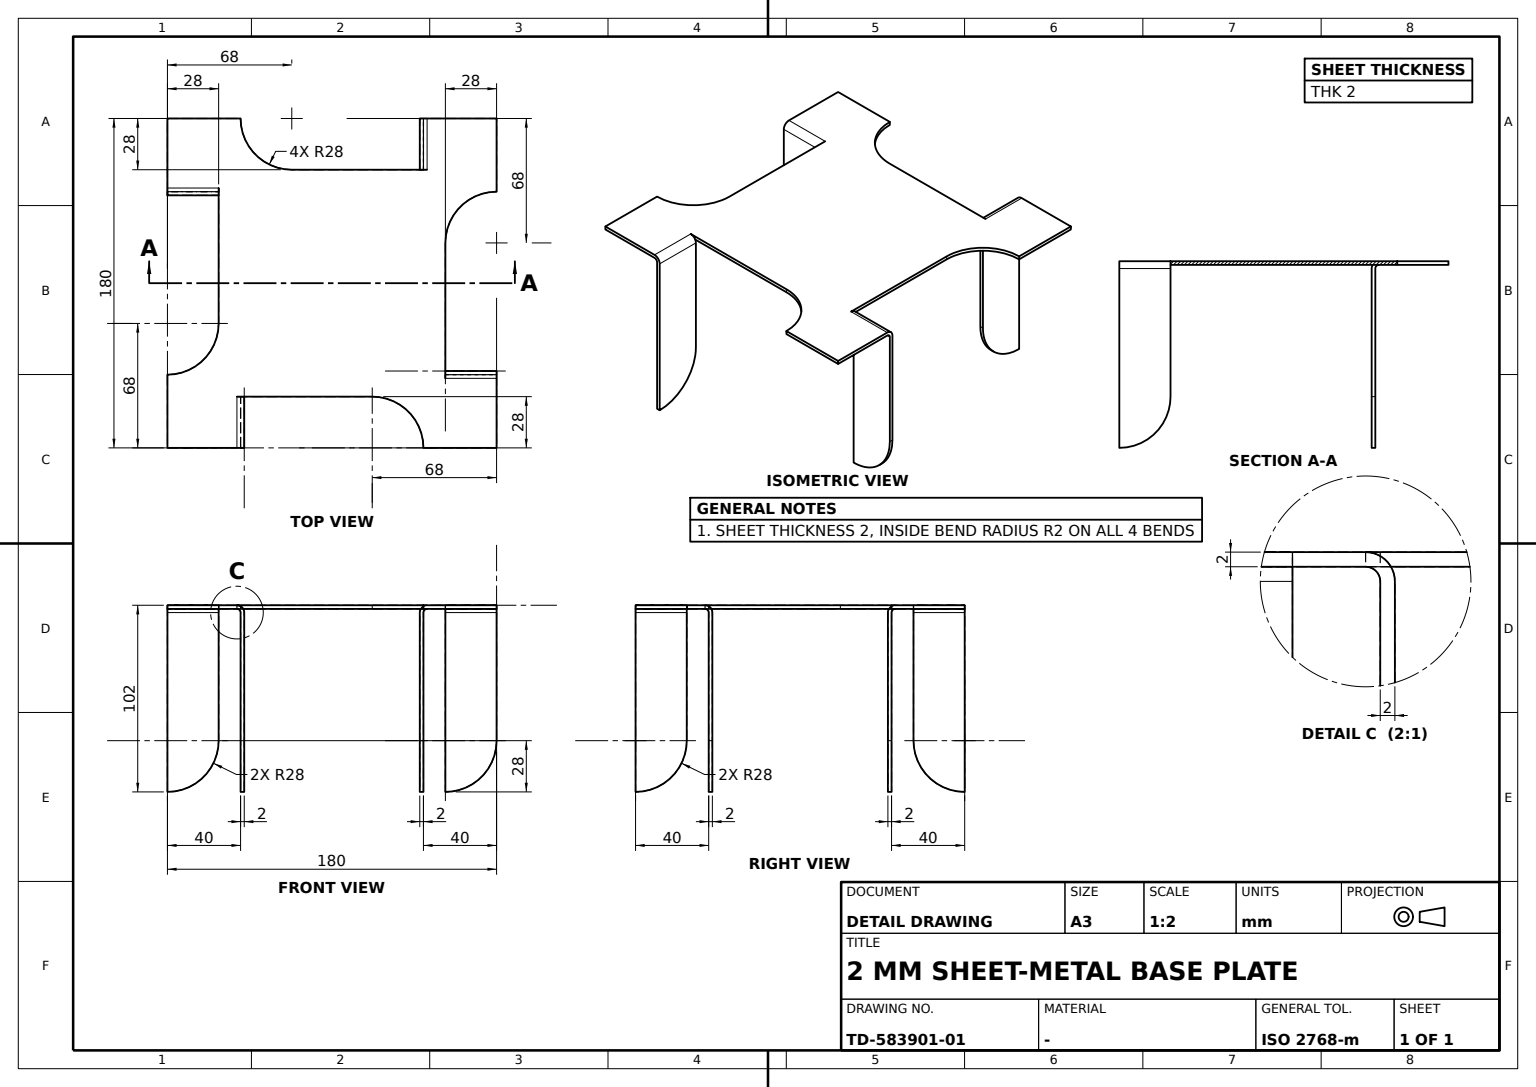
ISO-10303-21;
HEADER;
FILE_DESCRIPTION((''),'2;1');
FILE_NAME('','',(''),(''),'','','');
FILE_SCHEMA(('AUTOMOTIVE_DESIGN'));
ENDSEC;
DATA;
#1=APPLICATION_CONTEXT('');
#2=PRODUCT_CONTEXT('',#1,'mechanical');
#3=PRODUCT('','','',(#2));
#4=PRODUCT_DEFINITION_FORMATION('','',#3);
#5=PRODUCT_DEFINITION_CONTEXT('',#1,'design');
#6=PRODUCT_DEFINITION('','',#4,#5);
#7=PRODUCT_DEFINITION_SHAPE('','',#6);
#8=(LENGTH_UNIT()NAMED_UNIT(*)SI_UNIT(.MILLI.,.METRE.));
#9=(NAMED_UNIT(*)PLANE_ANGLE_UNIT()SI_UNIT($,.RADIAN.));
#10=(NAMED_UNIT(*)SI_UNIT($,.STERADIAN.)SOLID_ANGLE_UNIT());
#11=UNCERTAINTY_MEASURE_WITH_UNIT(LENGTH_MEASURE(0.005),#8,'distance_accuracy_value','');
#12=(GEOMETRIC_REPRESENTATION_CONTEXT(3)GLOBAL_UNCERTAINTY_ASSIGNED_CONTEXT((#11))GLOBAL_UNIT_ASSIGNED_CONTEXT((#8,#9,#10))REPRESENTATION_CONTEXT('',''));
#13=CARTESIAN_POINT('',(-62.,50.,-3.));
#14=VERTEX_POINT('',#13);
#15=CARTESIAN_POINT('',(-90.,50.,-3.));
#16=VERTEX_POINT('',#15);
#17=CARTESIAN_POINT('',(0.,50.,-3.));
#18=DIRECTION('',(-1.,0.,0.));
#19=VECTOR('',#18,1000.);
#20=LINE('',#17,#19);
#21=EDGE_CURVE('',#14,#16,#20,.T.);
#22=ORIENTED_EDGE('',*,*,#21,.T.);
#23=CARTESIAN_POINT('',(-90.,52.,-1.));
#24=VERTEX_POINT('',#23);
#25=CARTESIAN_POINT('',(-90.,52.,-3.));
#26=DIRECTION('',(1.,0.,0.));
#27=DIRECTION('',(0.,0.,-1.));
#28=AXIS2_PLACEMENT_3D('',#25,#26,#27);
#29=CIRCLE('',#28,2.);
#30=EDGE_CURVE('',#16,#24,#29,.F.);
#31=ORIENTED_EDGE('',*,*,#30,.T.);
#32=CARTESIAN_POINT('',(-62.,52.,-1.));
#33=VERTEX_POINT('',#32);
#34=CARTESIAN_POINT('',(0.,52.,-1.));
#35=LINE('',#34,#19);
#36=EDGE_CURVE('',#33,#24,#35,.T.);
#37=ORIENTED_EDGE('',*,*,#36,.F.);
#38=CARTESIAN_POINT('',(-62.,52.,-3.));
#39=AXIS2_PLACEMENT_3D('',#38,#26,#27);
#40=CIRCLE('',#39,2.);
#41=EDGE_CURVE('',#33,#14,#40,.T.);
#42=ORIENTED_EDGE('',*,*,#41,.T.);
#43=EDGE_LOOP('',(#22,#31,#37,#42));
#44=FACE_BOUND('',#43,.T.);
#45=CARTESIAN_POINT('',(0.,52.,-3.));
#46=DIRECTION('',(0.,0.,1.));
#47=AXIS2_PLACEMENT_3D('',#45,#18,#46);
#48=CYLINDRICAL_SURFACE('',#47,2.);
#49=ADVANCED_FACE('',(#44),#48,.F.);
#50=CARTESIAN_POINT('',(50.,90.,-101.));
#51=VERTEX_POINT('',#50);
#52=CARTESIAN_POINT('',(50.,62.,-73.));
#53=VERTEX_POINT('',#52);
#54=CARTESIAN_POINT('',(50.,90.,-73.));
#55=AXIS2_PLACEMENT_3D('',#54,#18,#46);
#56=CIRCLE('',#55,28.);
#57=EDGE_CURVE('',#51,#53,#56,.T.);
#58=ORIENTED_EDGE('',*,*,#57,.T.);
#59=CARTESIAN_POINT('',(48.,62.,-73.));
#60=VERTEX_POINT('',#59);
#61=LINE('',#52,#19);
#62=EDGE_CURVE('',#53,#60,#61,.T.);
#63=ORIENTED_EDGE('',*,*,#62,.T.);
#64=CARTESIAN_POINT('',(48.,90.,-101.));
#65=VERTEX_POINT('',#64);
#66=CARTESIAN_POINT('',(48.,90.,-73.));
#67=AXIS2_PLACEMENT_3D('',#66,#18,#46);
#68=CIRCLE('',#67,28.);
#69=EDGE_CURVE('',#65,#60,#68,.T.);
#70=ORIENTED_EDGE('',*,*,#69,.F.);
#71=LINE('',#50,#19);
#72=EDGE_CURVE('',#51,#65,#71,.T.);
#73=ORIENTED_EDGE('',*,*,#72,.F.);
#74=EDGE_LOOP('',(#58,#63,#70,#73));
#75=FACE_BOUND('',#74,.T.);
#76=DIRECTION('',(0.,1.,0.));
#77=AXIS2_PLACEMENT_3D('',#54,#18,#76);
#78=CYLINDRICAL_SURFACE('',#77,28.);
#79=ADVANCED_FACE('',(#75),#78,.T.);
#80=CARTESIAN_POINT('',(62.,-52.,1.));
#81=VERTEX_POINT('',#80);
#82=CARTESIAN_POINT('',(62.,-48.,-3.));
#83=VERTEX_POINT('',#82);
#84=CARTESIAN_POINT('',(62.,-52.,-3.));
#85=AXIS2_PLACEMENT_3D('',#84,#18,#46);
#86=CIRCLE('',#85,4.);
#87=EDGE_CURVE('',#81,#83,#86,.T.);
#88=ORIENTED_EDGE('',*,*,#87,.T.);
#89=CARTESIAN_POINT('',(62.,-48.,-101.));
#90=VERTEX_POINT('',#89);
#91=CARTESIAN_POINT('',(62.,-48.,-52.));
#92=VECTOR('',#27,1000.);
#93=LINE('',#91,#92);
#94=EDGE_CURVE('',#83,#90,#93,.T.);
#95=ORIENTED_EDGE('',*,*,#94,.T.);
#96=CARTESIAN_POINT('',(62.,-50.,-101.));
#97=VERTEX_POINT('',#96);
#98=VECTOR('',#76,1000.);
#99=LINE('',#96,#98);
#100=EDGE_CURVE('',#97,#90,#99,.T.);
#101=ORIENTED_EDGE('',*,*,#100,.F.);
#102=CARTESIAN_POINT('',(62.,-50.,-3.));
#103=VERTEX_POINT('',#102);
#104=CARTESIAN_POINT('',(62.,-50.,-52.));
#105=LINE('',#104,#92);
#106=EDGE_CURVE('',#103,#97,#105,.T.);
#107=ORIENTED_EDGE('',*,*,#106,.F.);
#108=CARTESIAN_POINT('',(62.,-52.,-1.));
#109=VERTEX_POINT('',#108);
#110=CIRCLE('',#85,2.);
#111=EDGE_CURVE('',#109,#103,#110,.T.);
#112=ORIENTED_EDGE('',*,*,#111,.F.);
#113=CARTESIAN_POINT('',(62.,-52.,-52.));
#114=LINE('',#113,#92);
#115=EDGE_CURVE('',#109,#81,#114,.F.);
#116=ORIENTED_EDGE('',*,*,#115,.T.);
#117=EDGE_LOOP('',(#88,#95,#101,#107,#112,#116));
#118=FACE_BOUND('',#117,.T.);
#119=AXIS2_PLACEMENT_3D('',#91,#18,#76);
#120=PLANE('',#119);
#121=ADVANCED_FACE('',(#118),#120,.T.);
#122=CARTESIAN_POINT('',(50.,-90.,1.));
#123=VERTEX_POINT('',#122);
#124=CARTESIAN_POINT('',(22.,-62.,1.));
#125=VERTEX_POINT('',#124);
#126=CARTESIAN_POINT('',(22.,-90.,1.));
#127=AXIS2_PLACEMENT_3D('',#126,#46,#26);
#128=CIRCLE('',#127,28.);
#129=EDGE_CURVE('',#123,#125,#128,.T.);
#130=ORIENTED_EDGE('',*,*,#129,.T.);
#131=CARTESIAN_POINT('',(22.,-62.,-1.));
#132=VERTEX_POINT('',#131);
#133=VECTOR('',#46,1000.);
#134=LINE('',#131,#133);
#135=EDGE_CURVE('',#132,#125,#134,.T.);
#136=ORIENTED_EDGE('',*,*,#135,.F.);
#137=CARTESIAN_POINT('',(50.,-90.,-1.));
#138=VERTEX_POINT('',#137);
#139=CARTESIAN_POINT('',(22.,-90.,-1.));
#140=AXIS2_PLACEMENT_3D('',#139,#46,#26);
#141=CIRCLE('',#140,28.);
#142=EDGE_CURVE('',#138,#132,#141,.T.);
#143=ORIENTED_EDGE('',*,*,#142,.F.);
#144=LINE('',#137,#133);
#145=EDGE_CURVE('',#138,#123,#144,.T.);
#146=ORIENTED_EDGE('',*,*,#145,.T.);
#147=EDGE_LOOP('',(#130,#136,#143,#146));
#148=FACE_BOUND('',#147,.T.);
#149=CYLINDRICAL_SURFACE('',#140,28.);
#150=ADVANCED_FACE('',(#148),#149,.F.);
#151=CARTESIAN_POINT('',(52.,62.,-1.));
#152=VERTEX_POINT('',#151);
#153=CARTESIAN_POINT('',(50.,62.,-3.));
#154=VERTEX_POINT('',#153);
#155=CARTESIAN_POINT('',(52.,62.,-3.));
#156=AXIS2_PLACEMENT_3D('',#155,#76,#46);
#157=CIRCLE('',#156,2.);
#158=EDGE_CURVE('',#152,#154,#157,.F.);
#159=ORIENTED_EDGE('',*,*,#158,.T.);
#160=CARTESIAN_POINT('',(50.,90.,-3.));
#161=VERTEX_POINT('',#160);
#162=CARTESIAN_POINT('',(50.,0.,-3.));
#163=LINE('',#162,#98);
#164=EDGE_CURVE('',#154,#161,#163,.T.);
#165=ORIENTED_EDGE('',*,*,#164,.T.);
#166=CARTESIAN_POINT('',(52.,90.,-1.));
#167=VERTEX_POINT('',#166);
#168=CARTESIAN_POINT('',(52.,90.,-3.));
#169=DIRECTION('',(0.,-1.,0.));
#170=AXIS2_PLACEMENT_3D('',#168,#169,#27);
#171=CIRCLE('',#170,2.);
#172=EDGE_CURVE('',#161,#167,#171,.F.);
#173=ORIENTED_EDGE('',*,*,#172,.T.);
#174=CARTESIAN_POINT('',(52.,0.,-1.));
#175=LINE('',#174,#98);
#176=EDGE_CURVE('',#152,#167,#175,.T.);
#177=ORIENTED_EDGE('',*,*,#176,.F.);
#178=EDGE_LOOP('',(#159,#165,#173,#177));
#179=FACE_BOUND('',#178,.T.);
#180=CARTESIAN_POINT('',(52.,0.,-3.));
#181=AXIS2_PLACEMENT_3D('',#180,#76,#46);
#182=CYLINDRICAL_SURFACE('',#181,2.);
#183=ADVANCED_FACE('',(#179),#182,.F.);
#184=CARTESIAN_POINT('',(62.,22.,-1.));
#185=VERTEX_POINT('',#184);
#186=CARTESIAN_POINT('',(62.,22.,1.));
#187=VERTEX_POINT('',#186);
#188=LINE('',#184,#133);
#189=EDGE_CURVE('',#185,#187,#188,.T.);
#190=ORIENTED_EDGE('',*,*,#189,.T.);
#191=CARTESIAN_POINT('',(62.,-48.,1.));
#192=LINE('',#191,#98);
#193=EDGE_CURVE('',#187,#81,#192,.F.);
#194=ORIENTED_EDGE('',*,*,#193,.T.);
#195=ORIENTED_EDGE('',*,*,#115,.F.);
#196=CARTESIAN_POINT('',(62.,-48.,-1.));
#197=LINE('',#196,#98);
#198=EDGE_CURVE('',#185,#109,#197,.F.);
#199=ORIENTED_EDGE('',*,*,#198,.F.);
#200=EDGE_LOOP('',(#190,#194,#195,#199));
#201=FACE_BOUND('',#200,.T.);
#202=ADVANCED_FACE('',(#201),#120,.F.);
#203=CARTESIAN_POINT('',(90.,50.,-1.));
#204=VERTEX_POINT('',#203);
#205=CARTESIAN_POINT('',(90.,50.,1.));
#206=VERTEX_POINT('',#205);
#207=LINE('',#203,#133);
#208=EDGE_CURVE('',#204,#206,#207,.T.);
#209=ORIENTED_EDGE('',*,*,#208,.T.);
#210=CARTESIAN_POINT('',(90.,22.,1.));
#211=AXIS2_PLACEMENT_3D('',#210,#46,#26);
#212=CIRCLE('',#211,28.);
#213=EDGE_CURVE('',#206,#187,#212,.T.);
#214=ORIENTED_EDGE('',*,*,#213,.T.);
#215=ORIENTED_EDGE('',*,*,#189,.F.);
#216=CARTESIAN_POINT('',(90.,22.,-1.));
#217=AXIS2_PLACEMENT_3D('',#216,#46,#26);
#218=CIRCLE('',#217,28.);
#219=EDGE_CURVE('',#204,#185,#218,.T.);
#220=ORIENTED_EDGE('',*,*,#219,.F.);
#221=EDGE_LOOP('',(#209,#214,#215,#220));
#222=FACE_BOUND('',#221,.T.);
#223=CYLINDRICAL_SURFACE('',#217,28.);
#224=ADVANCED_FACE('',(#222),#223,.F.);
#225=CARTESIAN_POINT('',(-62.,-22.,-1.));
#226=VERTEX_POINT('',#225);
#227=CARTESIAN_POINT('',(-62.,-22.,1.));
#228=VERTEX_POINT('',#227);
#229=LINE('',#225,#133);
#230=EDGE_CURVE('',#226,#228,#229,.T.);
#231=ORIENTED_EDGE('',*,*,#230,.T.);
#232=CARTESIAN_POINT('',(-62.,52.,1.));
#233=VERTEX_POINT('',#232);
#234=CARTESIAN_POINT('',(-62.,0.,1.));
#235=LINE('',#234,#98);
#236=EDGE_CURVE('',#228,#233,#235,.T.);
#237=ORIENTED_EDGE('',*,*,#236,.T.);
#238=CARTESIAN_POINT('',(-62.,52.,-52.));
#239=LINE('',#238,#133);
#240=EDGE_CURVE('',#33,#233,#239,.T.);
#241=ORIENTED_EDGE('',*,*,#240,.F.);
#242=CARTESIAN_POINT('',(-62.,0.,-1.));
#243=LINE('',#242,#98);
#244=EDGE_CURVE('',#33,#226,#243,.F.);
#245=ORIENTED_EDGE('',*,*,#244,.T.);
#246=EDGE_LOOP('',(#231,#237,#241,#245));
#247=FACE_BOUND('',#246,.T.);
#248=CARTESIAN_POINT('',(-62.,48.,-52.));
#249=AXIS2_PLACEMENT_3D('',#248,#26,#76);
#250=PLANE('',#249);
#251=ADVANCED_FACE('',(#247),#250,.F.);
#252=ORIENTED_EDGE('',*,*,#62,.F.);
#253=LINE('',#153,#133);
#254=EDGE_CURVE('',#154,#53,#253,.F.);
#255=ORIENTED_EDGE('',*,*,#254,.F.);
#256=ORIENTED_EDGE('',*,*,#158,.F.);
#257=CARTESIAN_POINT('',(52.,62.,1.));
#258=VERTEX_POINT('',#257);
#259=LINE('',#151,#133);
#260=EDGE_CURVE('',#152,#258,#259,.T.);
#261=ORIENTED_EDGE('',*,*,#260,.T.);
#262=CARTESIAN_POINT('',(48.,62.,-3.));
#263=VERTEX_POINT('',#262);
#264=CIRCLE('',#156,4.);
#265=EDGE_CURVE('',#258,#263,#264,.F.);
#266=ORIENTED_EDGE('',*,*,#265,.T.);
#267=CARTESIAN_POINT('',(48.,62.,-1.));
#268=LINE('',#267,#92);
#269=EDGE_CURVE('',#60,#263,#268,.F.);
#270=ORIENTED_EDGE('',*,*,#269,.F.);
#271=EDGE_LOOP('',(#252,#255,#256,#261,#266,#270));
#272=FACE_BOUND('',#271,.T.);
#273=DIRECTION('',(0.382683432,0.,0.923879533));
#274=AXIS2_PLACEMENT_3D('',#262,#76,#273);
#275=PLANE('',#274);
#276=ADVANCED_FACE('',(#272),#275,.F.);
#277=ORIENTED_EDGE('',*,*,#41,.F.);
#278=ORIENTED_EDGE('',*,*,#240,.T.);
#279=CARTESIAN_POINT('',(-62.,48.,-3.));
#280=VERTEX_POINT('',#279);
#281=CIRCLE('',#39,4.);
#282=EDGE_CURVE('',#233,#280,#281,.T.);
#283=ORIENTED_EDGE('',*,*,#282,.T.);
#284=CARTESIAN_POINT('',(-62.,48.,-73.));
#285=VERTEX_POINT('',#284);
#286=CARTESIAN_POINT('',(-62.,48.,-1.));
#287=LINE('',#286,#133);
#288=EDGE_CURVE('',#285,#280,#287,.T.);
#289=ORIENTED_EDGE('',*,*,#288,.F.);
#290=CARTESIAN_POINT('',(-62.,50.,-73.));
#291=VERTEX_POINT('',#290);
#292=VECTOR('',#169,1000.);
#293=LINE('',#290,#292);
#294=EDGE_CURVE('',#291,#285,#293,.T.);
#295=ORIENTED_EDGE('',*,*,#294,.F.);
#296=CARTESIAN_POINT('',(-62.,50.,-52.));
#297=LINE('',#296,#92);
#298=EDGE_CURVE('',#14,#291,#297,.T.);
#299=ORIENTED_EDGE('',*,*,#298,.F.);
#300=EDGE_LOOP('',(#277,#278,#283,#289,#295,#299));
#301=FACE_BOUND('',#300,.T.);
#302=ADVANCED_FACE('',(#301),#250,.T.);
#303=CARTESIAN_POINT('',(48.,90.,-3.));
#304=VERTEX_POINT('',#303);
#305=CARTESIAN_POINT('',(48.,0.,-3.));
#306=LINE('',#305,#98);
#307=EDGE_CURVE('',#263,#304,#306,.T.);
#308=ORIENTED_EDGE('',*,*,#307,.T.);
#309=CARTESIAN_POINT('',(48.,90.,-52.));
#310=LINE('',#309,#92);
#311=EDGE_CURVE('',#304,#65,#310,.T.);
#312=ORIENTED_EDGE('',*,*,#311,.T.);
#313=ORIENTED_EDGE('',*,*,#69,.T.);
#314=ORIENTED_EDGE('',*,*,#269,.T.);
#315=EDGE_LOOP('',(#308,#312,#313,#314));
#316=FACE_BOUND('',#315,.T.);
#317=CARTESIAN_POINT('',(48.,76.,-1.));
#318=AXIS2_PLACEMENT_3D('',#317,#18,#76);
#319=PLANE('',#318);
#320=ADVANCED_FACE('',(#316),#319,.T.);
#321=CARTESIAN_POINT('',(90.,-48.,-73.));
#322=VERTEX_POINT('',#321);
#323=CARTESIAN_POINT('',(62.,-48.,-73.));
#324=AXIS2_PLACEMENT_3D('',#323,#76,#46);
#325=CIRCLE('',#324,28.);
#326=EDGE_CURVE('',#322,#90,#325,.T.);
#327=ORIENTED_EDGE('',*,*,#326,.F.);
#328=CARTESIAN_POINT('',(90.,-50.,-73.));
#329=VERTEX_POINT('',#328);
#330=LINE('',#328,#98);
#331=EDGE_CURVE('',#329,#322,#330,.T.);
#332=ORIENTED_EDGE('',*,*,#331,.F.);
#333=CARTESIAN_POINT('',(62.,-50.,-73.));
#334=AXIS2_PLACEMENT_3D('',#333,#76,#46);
#335=CIRCLE('',#334,28.);
#336=EDGE_CURVE('',#329,#97,#335,.T.);
#337=ORIENTED_EDGE('',*,*,#336,.T.);
#338=ORIENTED_EDGE('',*,*,#100,.T.);
#339=EDGE_LOOP('',(#327,#332,#337,#338));
#340=FACE_BOUND('',#339,.T.);
#341=AXIS2_PLACEMENT_3D('',#333,#76,#26);
#342=CYLINDRICAL_SURFACE('',#341,28.);
#343=ADVANCED_FACE('',(#340),#342,.T.);
#344=ORIENTED_EDGE('',*,*,#145,.F.);
#345=CARTESIAN_POINT('',(90.,-90.,-1.));
#346=VERTEX_POINT('',#345);
#347=CARTESIAN_POINT('',(-90.,-90.,-1.));
#348=LINE('',#347,#19);
#349=EDGE_CURVE('',#346,#138,#348,.T.);
#350=ORIENTED_EDGE('',*,*,#349,.F.);
#351=CARTESIAN_POINT('',(90.,-90.,1.));
#352=VERTEX_POINT('',#351);
#353=CARTESIAN_POINT('',(90.,-90.,-52.));
#354=LINE('',#353,#133);
#355=EDGE_CURVE('',#352,#346,#354,.F.);
#356=ORIENTED_EDGE('',*,*,#355,.F.);
#357=CARTESIAN_POINT('',(-90.,-90.,1.));
#358=LINE('',#357,#19);
#359=EDGE_CURVE('',#352,#123,#358,.T.);
#360=ORIENTED_EDGE('',*,*,#359,.T.);
#361=EDGE_LOOP('',(#344,#350,#356,#360));
#362=FACE_BOUND('',#361,.T.);
#363=AXIS2_PLACEMENT_3D('',#347,#169,#26);
#364=PLANE('',#363);
#365=ADVANCED_FACE('',(#362),#364,.T.);
#366=CARTESIAN_POINT('',(-90.,48.,-3.));
#367=VERTEX_POINT('',#366);
#368=CARTESIAN_POINT('',(-90.,48.,-101.));
#369=VERTEX_POINT('',#368);
#370=CARTESIAN_POINT('',(-90.,48.,1.));
#371=LINE('',#370,#92);
#372=EDGE_CURVE('',#367,#369,#371,.T.);
#373=ORIENTED_EDGE('',*,*,#372,.F.);
#374=CARTESIAN_POINT('',(-90.,52.,1.));
#375=VERTEX_POINT('',#374);
#376=CIRCLE('',#28,4.);
#377=EDGE_CURVE('',#367,#375,#376,.F.);
#378=ORIENTED_EDGE('',*,*,#377,.T.);
#379=CARTESIAN_POINT('',(-90.,90.,1.));
#380=VERTEX_POINT('',#379);
#381=CARTESIAN_POINT('',(-90.,0.,1.));
#382=LINE('',#381,#98);
#383=EDGE_CURVE('',#380,#375,#382,.F.);
#384=ORIENTED_EDGE('',*,*,#383,.F.);
#385=CARTESIAN_POINT('',(-90.,90.,-1.));
#386=VERTEX_POINT('',#385);
#387=LINE('',#379,#92);
#388=EDGE_CURVE('',#380,#386,#387,.T.);
#389=ORIENTED_EDGE('',*,*,#388,.T.);
#390=CARTESIAN_POINT('',(-90.,0.,-1.));
#391=LINE('',#390,#98);
#392=EDGE_CURVE('',#386,#24,#391,.F.);
#393=ORIENTED_EDGE('',*,*,#392,.T.);
#394=ORIENTED_EDGE('',*,*,#30,.F.);
#395=CARTESIAN_POINT('',(-90.,50.,-101.));
#396=VERTEX_POINT('',#395);
#397=CARTESIAN_POINT('',(-90.,50.,1.));
#398=LINE('',#397,#92);
#399=EDGE_CURVE('',#16,#396,#398,.T.);
#400=ORIENTED_EDGE('',*,*,#399,.T.);
#401=LINE('',#395,#292);
#402=EDGE_CURVE('',#396,#369,#401,.T.);
#403=ORIENTED_EDGE('',*,*,#402,.T.);
#404=EDGE_LOOP('',(#373,#378,#384,#389,#393,#394,#400,#403));
#405=FACE_BOUND('',#404,.T.);
#406=DIRECTION('',(0.,-0.923879533,-0.382683432));
#407=AXIS2_PLACEMENT_3D('',#374,#26,#406);
#408=PLANE('',#407);
#409=ADVANCED_FACE('',(#405),#408,.F.);
#410=CARTESIAN_POINT('',(-48.,-90.,-101.));
#411=VERTEX_POINT('',#410);
#412=CARTESIAN_POINT('',(-48.,-90.,-3.));
#413=VERTEX_POINT('',#412);
#414=CARTESIAN_POINT('',(-48.,-90.,-1.));
#415=LINE('',#414,#92);
#416=EDGE_CURVE('',#411,#413,#415,.F.);
#417=ORIENTED_EDGE('',*,*,#416,.F.);
#418=CARTESIAN_POINT('',(-48.,-62.,-73.));
#419=VERTEX_POINT('',#418);
#420=CARTESIAN_POINT('',(-48.,-90.,-73.));
#421=AXIS2_PLACEMENT_3D('',#420,#26,#27);
#422=CIRCLE('',#421,28.);
#423=EDGE_CURVE('',#411,#419,#422,.T.);
#424=ORIENTED_EDGE('',*,*,#423,.T.);
#425=CARTESIAN_POINT('',(-48.,-62.,-3.));
#426=VERTEX_POINT('',#425);
#427=CARTESIAN_POINT('',(-48.,-62.,-1.));
#428=LINE('',#427,#92);
#429=EDGE_CURVE('',#419,#426,#428,.F.);
#430=ORIENTED_EDGE('',*,*,#429,.T.);
#431=CARTESIAN_POINT('',(-48.,0.,-3.));
#432=LINE('',#431,#292);
#433=EDGE_CURVE('',#426,#413,#432,.T.);
#434=ORIENTED_EDGE('',*,*,#433,.T.);
#435=EDGE_LOOP('',(#417,#424,#430,#434));
#436=FACE_BOUND('',#435,.T.);
#437=CARTESIAN_POINT('',(-48.,-76.,-1.));
#438=AXIS2_PLACEMENT_3D('',#437,#26,#169);
#439=PLANE('',#438);
#440=ADVANCED_FACE('',(#436),#439,.T.);
#441=CARTESIAN_POINT('',(90.,90.,-1.));
#442=VERTEX_POINT('',#441);
#443=CARTESIAN_POINT('',(90.,-48.,-1.));
#444=LINE('',#443,#98);
#445=EDGE_CURVE('',#442,#204,#444,.F.);
#446=ORIENTED_EDGE('',*,*,#445,.F.);
#447=CARTESIAN_POINT('',(90.,90.,1.));
#448=VERTEX_POINT('',#447);
#449=CARTESIAN_POINT('',(90.,90.,-52.));
#450=LINE('',#449,#92);
#451=EDGE_CURVE('',#448,#442,#450,.T.);
#452=ORIENTED_EDGE('',*,*,#451,.F.);
#453=CARTESIAN_POINT('',(90.,-48.,1.));
#454=LINE('',#453,#98);
#455=EDGE_CURVE('',#448,#206,#454,.F.);
#456=ORIENTED_EDGE('',*,*,#455,.T.);
#457=ORIENTED_EDGE('',*,*,#208,.F.);
#458=EDGE_LOOP('',(#446,#452,#456,#457));
#459=FACE_BOUND('',#458,.T.);
#460=CARTESIAN_POINT('',(90.,-48.,-52.));
#461=AXIS2_PLACEMENT_3D('',#460,#18,#76);
#462=PLANE('',#461);
#463=ADVANCED_FACE('',(#459),#462,.F.);
#464=ORIENTED_EDGE('',*,*,#307,.F.);
#465=ORIENTED_EDGE('',*,*,#265,.F.);
#466=CARTESIAN_POINT('',(52.,90.,1.));
#467=VERTEX_POINT('',#466);
#468=CARTESIAN_POINT('',(52.,0.,1.));
#469=LINE('',#468,#98);
#470=EDGE_CURVE('',#258,#467,#469,.T.);
#471=ORIENTED_EDGE('',*,*,#470,.T.);
#472=CIRCLE('',#170,4.);
#473=EDGE_CURVE('',#304,#467,#472,.F.);
#474=ORIENTED_EDGE('',*,*,#473,.F.);
#475=EDGE_LOOP('',(#464,#465,#471,#474));
#476=FACE_BOUND('',#475,.T.);
#477=CYLINDRICAL_SURFACE('',#181,4.);
#478=ADVANCED_FACE('',(#476),#477,.T.);
#479=CARTESIAN_POINT('',(0.,52.,1.));
#480=LINE('',#479,#19);
#481=EDGE_CURVE('',#233,#375,#480,.T.);
#482=ORIENTED_EDGE('',*,*,#481,.T.);
#483=ORIENTED_EDGE('',*,*,#377,.F.);
#484=CARTESIAN_POINT('',(0.,48.,-3.));
#485=LINE('',#484,#19);
#486=EDGE_CURVE('',#280,#367,#485,.T.);
#487=ORIENTED_EDGE('',*,*,#486,.F.);
#488=ORIENTED_EDGE('',*,*,#282,.F.);
#489=EDGE_LOOP('',(#482,#483,#487,#488));
#490=FACE_BOUND('',#489,.T.);
#491=CYLINDRICAL_SURFACE('',#47,4.);
#492=ADVANCED_FACE('',(#490),#491,.T.);
#493=CARTESIAN_POINT('',(50.,90.,-52.));
#494=LINE('',#493,#92);
#495=EDGE_CURVE('',#161,#51,#494,.T.);
#496=ORIENTED_EDGE('',*,*,#495,.F.);
#497=ORIENTED_EDGE('',*,*,#164,.F.);
#498=ORIENTED_EDGE('',*,*,#254,.T.);
#499=ORIENTED_EDGE('',*,*,#57,.F.);
#500=EDGE_LOOP('',(#496,#497,#498,#499));
#501=FACE_BOUND('',#500,.T.);
#502=CARTESIAN_POINT('',(50.,76.,-1.));
#503=AXIS2_PLACEMENT_3D('',#502,#18,#76);
#504=PLANE('',#503);
#505=ADVANCED_FACE('',(#501),#504,.F.);
#506=CARTESIAN_POINT('',(-50.,-90.,-101.));
#507=VERTEX_POINT('',#506);
#508=CARTESIAN_POINT('',(-50.,-62.,-73.));
#509=VERTEX_POINT('',#508);
#510=CARTESIAN_POINT('',(-50.,-90.,-73.));
#511=AXIS2_PLACEMENT_3D('',#510,#26,#27);
#512=CIRCLE('',#511,28.);
#513=EDGE_CURVE('',#507,#509,#512,.T.);
#514=ORIENTED_EDGE('',*,*,#513,.F.);
#515=CARTESIAN_POINT('',(-50.,-90.,-3.));
#516=VERTEX_POINT('',#515);
#517=CARTESIAN_POINT('',(-50.,-90.,-1.));
#518=LINE('',#517,#92);
#519=EDGE_CURVE('',#507,#516,#518,.F.);
#520=ORIENTED_EDGE('',*,*,#519,.T.);
#521=CARTESIAN_POINT('',(-50.,-62.,-3.));
#522=VERTEX_POINT('',#521);
#523=CARTESIAN_POINT('',(-50.,0.,-3.));
#524=LINE('',#523,#292);
#525=EDGE_CURVE('',#522,#516,#524,.T.);
#526=ORIENTED_EDGE('',*,*,#525,.F.);
#527=CARTESIAN_POINT('',(-50.,-62.,-1.));
#528=LINE('',#527,#133);
#529=EDGE_CURVE('',#522,#509,#528,.F.);
#530=ORIENTED_EDGE('',*,*,#529,.T.);
#531=EDGE_LOOP('',(#514,#520,#526,#530));
#532=FACE_BOUND('',#531,.T.);
#533=CARTESIAN_POINT('',(-50.,-76.,-1.));
#534=AXIS2_PLACEMENT_3D('',#533,#26,#169);
#535=PLANE('',#534);
#536=ADVANCED_FACE('',(#532),#535,.F.);
#537=ORIENTED_EDGE('',*,*,#230,.F.);
#538=CARTESIAN_POINT('',(-90.,-50.,-1.));
#539=VERTEX_POINT('',#538);
#540=CARTESIAN_POINT('',(-90.,-22.,-1.));
#541=AXIS2_PLACEMENT_3D('',#540,#46,#26);
#542=CIRCLE('',#541,28.);
#543=EDGE_CURVE('',#539,#226,#542,.T.);
#544=ORIENTED_EDGE('',*,*,#543,.F.);
#545=CARTESIAN_POINT('',(-90.,-50.,1.));
#546=VERTEX_POINT('',#545);
#547=LINE('',#538,#133);
#548=EDGE_CURVE('',#539,#546,#547,.T.);
#549=ORIENTED_EDGE('',*,*,#548,.T.);
#550=CARTESIAN_POINT('',(-90.,-22.,1.));
#551=AXIS2_PLACEMENT_3D('',#550,#46,#26);
#552=CIRCLE('',#551,28.);
#553=EDGE_CURVE('',#546,#228,#552,.T.);
#554=ORIENTED_EDGE('',*,*,#553,.T.);
#555=EDGE_LOOP('',(#537,#544,#549,#554));
#556=FACE_BOUND('',#555,.T.);
#557=CYLINDRICAL_SURFACE('',#541,28.);
#558=ADVANCED_FACE('',(#556),#557,.F.);
#559=CARTESIAN_POINT('',(-52.,-62.,-1.));
#560=VERTEX_POINT('',#559);
#561=CARTESIAN_POINT('',(0.,-62.,-1.));
#562=VECTOR('',#26,1000.);
#563=LINE('',#561,#562);
#564=EDGE_CURVE('',#560,#132,#563,.T.);
#565=ORIENTED_EDGE('',*,*,#564,.T.);
#566=ORIENTED_EDGE('',*,*,#135,.T.);
#567=CARTESIAN_POINT('',(-52.,-62.,1.));
#568=VERTEX_POINT('',#567);
#569=CARTESIAN_POINT('',(0.,-62.,1.));
#570=LINE('',#569,#562);
#571=EDGE_CURVE('',#125,#568,#570,.F.);
#572=ORIENTED_EDGE('',*,*,#571,.T.);
#573=LINE('',#559,#133);
#574=EDGE_CURVE('',#560,#568,#573,.T.);
#575=ORIENTED_EDGE('',*,*,#574,.F.);
#576=EDGE_LOOP('',(#565,#566,#572,#575));
#577=FACE_BOUND('',#576,.T.);
#578=AXIS2_PLACEMENT_3D('',#527,#169,#26);
#579=PLANE('',#578);
#580=ADVANCED_FACE('',(#577),#579,.T.);
#581=ORIENTED_EDGE('',*,*,#288,.T.);
#582=ORIENTED_EDGE('',*,*,#486,.T.);
#583=ORIENTED_EDGE('',*,*,#372,.T.);
#584=CARTESIAN_POINT('',(-90.,48.,-73.));
#585=AXIS2_PLACEMENT_3D('',#584,#169,#27);
#586=CIRCLE('',#585,28.);
#587=EDGE_CURVE('',#369,#285,#586,.T.);
#588=ORIENTED_EDGE('',*,*,#587,.T.);
#589=EDGE_LOOP('',(#581,#582,#583,#588));
#590=FACE_BOUND('',#589,.T.);
#591=CARTESIAN_POINT('',(-76.,48.,-1.));
#592=AXIS2_PLACEMENT_3D('',#591,#169,#18);
#593=PLANE('',#592);
#594=ADVANCED_FACE('',(#590),#593,.T.);
#595=CARTESIAN_POINT('',(-22.,62.,-1.));
#596=VERTEX_POINT('',#595);
#597=CARTESIAN_POINT('',(-22.,62.,1.));
#598=VERTEX_POINT('',#597);
#599=LINE('',#595,#133);
#600=EDGE_CURVE('',#596,#598,#599,.T.);
#601=ORIENTED_EDGE('',*,*,#600,.T.);
#602=CARTESIAN_POINT('',(48.,62.,1.));
#603=LINE('',#602,#562);
#604=EDGE_CURVE('',#598,#258,#603,.T.);
#605=ORIENTED_EDGE('',*,*,#604,.T.);
#606=ORIENTED_EDGE('',*,*,#260,.F.);
#607=CARTESIAN_POINT('',(0.,62.,-1.));
#608=LINE('',#607,#19);
#609=EDGE_CURVE('',#152,#596,#608,.T.);
#610=ORIENTED_EDGE('',*,*,#609,.T.);
#611=EDGE_LOOP('',(#601,#605,#606,#610));
#612=FACE_BOUND('',#611,.T.);
#613=ADVANCED_FACE('',(#612),#275,.T.);
#614=ORIENTED_EDGE('',*,*,#548,.F.);
#615=VERTEX_POINT('',#347);
#616=LINE('',#23,#292);
#617=EDGE_CURVE('',#615,#539,#616,.F.);
#618=ORIENTED_EDGE('',*,*,#617,.F.);
#619=VERTEX_POINT('',#357);
#620=LINE('',#347,#133);
#621=EDGE_CURVE('',#619,#615,#620,.F.);
#622=ORIENTED_EDGE('',*,*,#621,.F.);
#623=LINE('',#374,#292);
#624=EDGE_CURVE('',#619,#546,#623,.F.);
#625=ORIENTED_EDGE('',*,*,#624,.T.);
#626=EDGE_LOOP('',(#614,#618,#622,#625));
#627=FACE_BOUND('',#626,.T.);
#628=ADVANCED_FACE('',(#627),#408,.F.);
#629=CARTESIAN_POINT('',(-90.,50.,-73.));
#630=AXIS2_PLACEMENT_3D('',#629,#169,#27);
#631=CIRCLE('',#630,28.);
#632=EDGE_CURVE('',#396,#291,#631,.T.);
#633=ORIENTED_EDGE('',*,*,#632,.F.);
#634=ORIENTED_EDGE('',*,*,#399,.F.);
#635=ORIENTED_EDGE('',*,*,#21,.F.);
#636=ORIENTED_EDGE('',*,*,#298,.T.);
#637=EDGE_LOOP('',(#633,#634,#635,#636));
#638=FACE_BOUND('',#637,.T.);
#639=CARTESIAN_POINT('',(-76.,50.,-1.));
#640=AXIS2_PLACEMENT_3D('',#639,#169,#18);
#641=PLANE('',#640);
#642=ADVANCED_FACE('',(#638),#641,.F.);
#643=CARTESIAN_POINT('',(-52.,-62.,-3.));
#644=AXIS2_PLACEMENT_3D('',#643,#169,#27);
#645=CIRCLE('',#644,2.);
#646=EDGE_CURVE('',#560,#522,#645,.F.);
#647=ORIENTED_EDGE('',*,*,#646,.F.);
#648=ORIENTED_EDGE('',*,*,#574,.T.);
#649=CIRCLE('',#644,4.);
#650=EDGE_CURVE('',#568,#426,#649,.F.);
#651=ORIENTED_EDGE('',*,*,#650,.T.);
#652=ORIENTED_EDGE('',*,*,#429,.F.);
#653=LINE('',#508,#562);
#654=EDGE_CURVE('',#509,#419,#653,.T.);
#655=ORIENTED_EDGE('',*,*,#654,.F.);
#656=ORIENTED_EDGE('',*,*,#529,.F.);
#657=EDGE_LOOP('',(#647,#648,#651,#652,#655,#656));
#658=FACE_BOUND('',#657,.T.);
#659=ADVANCED_FACE('',(#658),#579,.F.);
#660=CARTESIAN_POINT('',(-50.,90.,-1.));
#661=VERTEX_POINT('',#660);
#662=CARTESIAN_POINT('',(48.,90.,-1.));
#663=LINE('',#662,#19);
#664=EDGE_CURVE('',#386,#661,#663,.F.);
#665=ORIENTED_EDGE('',*,*,#664,.F.);
#666=ORIENTED_EDGE('',*,*,#388,.F.);
#667=CARTESIAN_POINT('',(-50.,90.,1.));
#668=VERTEX_POINT('',#667);
#669=CARTESIAN_POINT('',(48.,90.,1.));
#670=LINE('',#669,#19);
#671=EDGE_CURVE('',#380,#668,#670,.F.);
#672=ORIENTED_EDGE('',*,*,#671,.T.);
#673=LINE('',#660,#133);
#674=EDGE_CURVE('',#661,#668,#673,.T.);
#675=ORIENTED_EDGE('',*,*,#674,.F.);
#676=EDGE_LOOP('',(#665,#666,#672,#675));
#677=FACE_BOUND('',#676,.T.);
#678=AXIS2_PLACEMENT_3D('',#309,#169,#26);
#679=PLANE('',#678);
#680=ADVANCED_FACE('',(#677),#679,.F.);
#681=LINE('',#506,#562);
#682=EDGE_CURVE('',#507,#411,#681,.T.);
#683=ORIENTED_EDGE('',*,*,#682,.F.);
#684=ORIENTED_EDGE('',*,*,#513,.T.);
#685=ORIENTED_EDGE('',*,*,#654,.T.);
#686=ORIENTED_EDGE('',*,*,#423,.F.);
#687=EDGE_LOOP('',(#683,#684,#685,#686));
#688=FACE_BOUND('',#687,.T.);
#689=AXIS2_PLACEMENT_3D('',#510,#26,#169);
#690=CYLINDRICAL_SURFACE('',#689,28.);
#691=ADVANCED_FACE('',(#688),#690,.T.);
#692=ORIENTED_EDGE('',*,*,#106,.T.);
#693=ORIENTED_EDGE('',*,*,#336,.F.);
#694=CARTESIAN_POINT('',(90.,-50.,-3.));
#695=VERTEX_POINT('',#694);
#696=CARTESIAN_POINT('',(90.,-50.,-52.));
#697=LINE('',#696,#92);
#698=EDGE_CURVE('',#695,#329,#697,.T.);
#699=ORIENTED_EDGE('',*,*,#698,.F.);
#700=CARTESIAN_POINT('',(0.,-50.,-3.));
#701=LINE('',#700,#562);
#702=EDGE_CURVE('',#103,#695,#701,.T.);
#703=ORIENTED_EDGE('',*,*,#702,.F.);
#704=EDGE_LOOP('',(#692,#693,#699,#703));
#705=FACE_BOUND('',#704,.T.);
#706=CARTESIAN_POINT('',(76.,-50.,-1.));
#707=AXIS2_PLACEMENT_3D('',#706,#76,#26);
#708=PLANE('',#707);
#709=ADVANCED_FACE('',(#705),#708,.F.);
#710=ORIENTED_EDGE('',*,*,#383,.T.);
#711=ORIENTED_EDGE('',*,*,#481,.F.);
#712=ORIENTED_EDGE('',*,*,#236,.F.);
#713=ORIENTED_EDGE('',*,*,#553,.F.);
#714=ORIENTED_EDGE('',*,*,#624,.F.);
#715=CARTESIAN_POINT('',(-52.,-90.,1.));
#716=VERTEX_POINT('',#715);
#717=CARTESIAN_POINT('',(0.,-90.,1.));
#718=LINE('',#717,#562);
#719=EDGE_CURVE('',#619,#716,#718,.T.);
#720=ORIENTED_EDGE('',*,*,#719,.T.);
#721=CARTESIAN_POINT('',(-52.,0.,1.));
#722=LINE('',#721,#292);
#723=EDGE_CURVE('',#568,#716,#722,.T.);
#724=ORIENTED_EDGE('',*,*,#723,.F.);
#725=ORIENTED_EDGE('',*,*,#571,.F.);
#726=ORIENTED_EDGE('',*,*,#129,.F.);
#727=ORIENTED_EDGE('',*,*,#359,.F.);
#728=CARTESIAN_POINT('',(90.,-52.,1.));
#729=VERTEX_POINT('',#728);
#730=CARTESIAN_POINT('',(90.,0.,1.));
#731=LINE('',#730,#292);
#732=EDGE_CURVE('',#352,#729,#731,.F.);
#733=ORIENTED_EDGE('',*,*,#732,.T.);
#734=CARTESIAN_POINT('',(0.,-52.,1.));
#735=LINE('',#734,#562);
#736=EDGE_CURVE('',#81,#729,#735,.T.);
#737=ORIENTED_EDGE('',*,*,#736,.F.);
#738=ORIENTED_EDGE('',*,*,#193,.F.);
#739=ORIENTED_EDGE('',*,*,#213,.F.);
#740=ORIENTED_EDGE('',*,*,#455,.F.);
#741=CARTESIAN_POINT('',(0.,90.,1.));
#742=LINE('',#741,#562);
#743=EDGE_CURVE('',#448,#467,#742,.F.);
#744=ORIENTED_EDGE('',*,*,#743,.T.);
#745=ORIENTED_EDGE('',*,*,#470,.F.);
#746=ORIENTED_EDGE('',*,*,#604,.F.);
#747=CARTESIAN_POINT('',(-22.,90.,1.));
#748=AXIS2_PLACEMENT_3D('',#747,#46,#26);
#749=CIRCLE('',#748,28.);
#750=EDGE_CURVE('',#668,#598,#749,.T.);
#751=ORIENTED_EDGE('',*,*,#750,.F.);
#752=ORIENTED_EDGE('',*,*,#671,.F.);
#753=EDGE_LOOP('',(#710,#711,#712,#713,#714,#720,#724,#725,#726,#727,#733,#737,#738,#739,#740,#744,#745,#746,#751,#752));
#754=FACE_BOUND('',#753,.T.);
#755=CARTESIAN_POINT('',(0.,0.,1.));
#756=AXIS2_PLACEMENT_3D('',#755,#46,#26);
#757=PLANE('',#756);
#758=ADVANCED_FACE('',(#754),#757,.T.);
#759=ORIENTED_EDGE('',*,*,#723,.T.);
#760=CARTESIAN_POINT('',(-52.,-90.,-3.));
#761=AXIS2_PLACEMENT_3D('',#760,#169,#27);
#762=CIRCLE('',#761,4.);
#763=EDGE_CURVE('',#413,#716,#762,.T.);
#764=ORIENTED_EDGE('',*,*,#763,.F.);
#765=ORIENTED_EDGE('',*,*,#433,.F.);
#766=ORIENTED_EDGE('',*,*,#650,.F.);
#767=EDGE_LOOP('',(#759,#764,#765,#766));
#768=FACE_BOUND('',#767,.T.);
#769=CARTESIAN_POINT('',(-52.,0.,-3.));
#770=AXIS2_PLACEMENT_3D('',#769,#169,#46);
#771=CYLINDRICAL_SURFACE('',#770,4.);
#772=ADVANCED_FACE('',(#768),#771,.T.);
#773=ORIENTED_EDGE('',*,*,#600,.F.);
#774=CARTESIAN_POINT('',(-22.,90.,-1.));
#775=AXIS2_PLACEMENT_3D('',#774,#46,#26);
#776=CIRCLE('',#775,28.);
#777=EDGE_CURVE('',#661,#596,#776,.T.);
#778=ORIENTED_EDGE('',*,*,#777,.F.);
#779=ORIENTED_EDGE('',*,*,#674,.T.);
#780=ORIENTED_EDGE('',*,*,#750,.T.);
#781=EDGE_LOOP('',(#773,#778,#779,#780));
#782=FACE_BOUND('',#781,.T.);
#783=CYLINDRICAL_SURFACE('',#775,28.);
#784=ADVANCED_FACE('',(#782),#783,.F.);
#785=ORIENTED_EDGE('',*,*,#732,.F.);
#786=ORIENTED_EDGE('',*,*,#355,.T.);
#787=CARTESIAN_POINT('',(90.,-52.,-1.));
#788=VERTEX_POINT('',#787);
#789=CARTESIAN_POINT('',(90.,0.,-1.));
#790=LINE('',#789,#292);
#791=EDGE_CURVE('',#346,#788,#790,.F.);
#792=ORIENTED_EDGE('',*,*,#791,.T.);
#793=CARTESIAN_POINT('',(90.,-52.,-3.));
#794=AXIS2_PLACEMENT_3D('',#793,#18,#46);
#795=CIRCLE('',#794,2.);
#796=EDGE_CURVE('',#695,#788,#795,.F.);
#797=ORIENTED_EDGE('',*,*,#796,.F.);
#798=ORIENTED_EDGE('',*,*,#698,.T.);
#799=ORIENTED_EDGE('',*,*,#331,.T.);
#800=CARTESIAN_POINT('',(90.,-48.,-3.));
#801=VERTEX_POINT('',#800);
#802=LINE('',#443,#133);
#803=EDGE_CURVE('',#322,#801,#802,.T.);
#804=ORIENTED_EDGE('',*,*,#803,.T.);
#805=CIRCLE('',#794,4.);
#806=EDGE_CURVE('',#801,#729,#805,.F.);
#807=ORIENTED_EDGE('',*,*,#806,.T.);
#808=EDGE_LOOP('',(#785,#786,#792,#797,#798,#799,#804,#807));
#809=FACE_BOUND('',#808,.T.);
#810=ADVANCED_FACE('',(#809),#462,.F.);
#811=CARTESIAN_POINT('',(0.,-48.,-3.));
#812=LINE('',#811,#562);
#813=EDGE_CURVE('',#83,#801,#812,.T.);
#814=ORIENTED_EDGE('',*,*,#813,.T.);
#815=ORIENTED_EDGE('',*,*,#803,.F.);
#816=ORIENTED_EDGE('',*,*,#326,.T.);
#817=ORIENTED_EDGE('',*,*,#94,.F.);
#818=EDGE_LOOP('',(#814,#815,#816,#817));
#819=FACE_BOUND('',#818,.T.);
#820=CARTESIAN_POINT('',(76.,-48.,-1.));
#821=AXIS2_PLACEMENT_3D('',#820,#76,#26);
#822=PLANE('',#821);
#823=ADVANCED_FACE('',(#819),#822,.T.);
#824=ORIENTED_EDGE('',*,*,#495,.T.);
#825=ORIENTED_EDGE('',*,*,#72,.T.);
#826=ORIENTED_EDGE('',*,*,#311,.F.);
#827=ORIENTED_EDGE('',*,*,#473,.T.);
#828=ORIENTED_EDGE('',*,*,#743,.F.);
#829=ORIENTED_EDGE('',*,*,#451,.T.);
#830=CARTESIAN_POINT('',(0.,90.,-1.));
#831=LINE('',#830,#562);
#832=EDGE_CURVE('',#442,#167,#831,.F.);
#833=ORIENTED_EDGE('',*,*,#832,.T.);
#834=ORIENTED_EDGE('',*,*,#172,.F.);
#835=EDGE_LOOP('',(#824,#825,#826,#827,#828,#829,#833,#834));
#836=FACE_BOUND('',#835,.T.);
#837=ADVANCED_FACE('',(#836),#679,.F.);
#838=ORIENTED_EDGE('',*,*,#111,.T.);
#839=ORIENTED_EDGE('',*,*,#702,.T.);
#840=ORIENTED_EDGE('',*,*,#796,.T.);
#841=CARTESIAN_POINT('',(0.,-52.,-1.));
#842=LINE('',#841,#562);
#843=EDGE_CURVE('',#109,#788,#842,.T.);
#844=ORIENTED_EDGE('',*,*,#843,.F.);
#845=EDGE_LOOP('',(#838,#839,#840,#844));
#846=FACE_BOUND('',#845,.T.);
#847=CARTESIAN_POINT('',(0.,-52.,-3.));
#848=AXIS2_PLACEMENT_3D('',#847,#26,#46);
#849=CYLINDRICAL_SURFACE('',#848,2.);
#850=ADVANCED_FACE('',(#846),#849,.F.);
#851=ORIENTED_EDGE('',*,*,#806,.F.);
#852=ORIENTED_EDGE('',*,*,#813,.F.);
#853=ORIENTED_EDGE('',*,*,#87,.F.);
#854=ORIENTED_EDGE('',*,*,#736,.T.);
#855=EDGE_LOOP('',(#851,#852,#853,#854));
#856=FACE_BOUND('',#855,.T.);
#857=CYLINDRICAL_SURFACE('',#848,4.);
#858=ADVANCED_FACE('',(#856),#857,.T.);
#859=CARTESIAN_POINT('',(-52.,-90.,-1.));
#860=VERTEX_POINT('',#859);
#861=CARTESIAN_POINT('',(-52.,0.,-1.));
#862=LINE('',#861,#292);
#863=EDGE_CURVE('',#560,#860,#862,.T.);
#864=ORIENTED_EDGE('',*,*,#863,.F.);
#865=ORIENTED_EDGE('',*,*,#646,.T.);
#866=ORIENTED_EDGE('',*,*,#525,.T.);
#867=CIRCLE('',#761,2.);
#868=EDGE_CURVE('',#516,#860,#867,.T.);
#869=ORIENTED_EDGE('',*,*,#868,.T.);
#870=EDGE_LOOP('',(#864,#865,#866,#869));
#871=FACE_BOUND('',#870,.T.);
#872=CYLINDRICAL_SURFACE('',#770,2.);
#873=ADVANCED_FACE('',(#871),#872,.F.);
#874=ORIENTED_EDGE('',*,*,#445,.T.);
#875=ORIENTED_EDGE('',*,*,#219,.T.);
#876=ORIENTED_EDGE('',*,*,#198,.T.);
#877=ORIENTED_EDGE('',*,*,#843,.T.);
#878=ORIENTED_EDGE('',*,*,#791,.F.);
#879=ORIENTED_EDGE('',*,*,#349,.T.);
#880=ORIENTED_EDGE('',*,*,#142,.T.);
#881=ORIENTED_EDGE('',*,*,#564,.F.);
#882=ORIENTED_EDGE('',*,*,#863,.T.);
#883=CARTESIAN_POINT('',(0.,-90.,-1.));
#884=LINE('',#883,#562);
#885=EDGE_CURVE('',#615,#860,#884,.T.);
#886=ORIENTED_EDGE('',*,*,#885,.F.);
#887=ORIENTED_EDGE('',*,*,#617,.T.);
#888=ORIENTED_EDGE('',*,*,#543,.T.);
#889=ORIENTED_EDGE('',*,*,#244,.F.);
#890=ORIENTED_EDGE('',*,*,#36,.T.);
#891=ORIENTED_EDGE('',*,*,#392,.F.);
#892=ORIENTED_EDGE('',*,*,#664,.T.);
#893=ORIENTED_EDGE('',*,*,#777,.T.);
#894=ORIENTED_EDGE('',*,*,#609,.F.);
#895=ORIENTED_EDGE('',*,*,#176,.T.);
#896=ORIENTED_EDGE('',*,*,#832,.F.);
#897=EDGE_LOOP('',(#874,#875,#876,#877,#878,#879,#880,#881,#882,#886,#887,#888,#889,#890,#891,#892,#893,#894,#895,#896));
#898=FACE_BOUND('',#897,.T.);
#899=CARTESIAN_POINT('',(0.,0.,-1.));
#900=AXIS2_PLACEMENT_3D('',#899,#46,#26);
#901=PLANE('',#900);
#902=ADVANCED_FACE('',(#898),#901,.F.);
#903=ORIENTED_EDGE('',*,*,#682,.T.);
#904=ORIENTED_EDGE('',*,*,#416,.T.);
#905=ORIENTED_EDGE('',*,*,#763,.T.);
#906=ORIENTED_EDGE('',*,*,#719,.F.);
#907=ORIENTED_EDGE('',*,*,#621,.T.);
#908=ORIENTED_EDGE('',*,*,#885,.T.);
#909=ORIENTED_EDGE('',*,*,#868,.F.);
#910=ORIENTED_EDGE('',*,*,#519,.F.);
#911=EDGE_LOOP('',(#903,#904,#905,#906,#907,#908,#909,#910));
#912=FACE_BOUND('',#911,.T.);
#913=ADVANCED_FACE('',(#912),#364,.T.);
#914=ORIENTED_EDGE('',*,*,#587,.F.);
#915=ORIENTED_EDGE('',*,*,#402,.F.);
#916=ORIENTED_EDGE('',*,*,#632,.T.);
#917=ORIENTED_EDGE('',*,*,#294,.T.);
#918=EDGE_LOOP('',(#914,#915,#916,#917));
#919=FACE_BOUND('',#918,.T.);
#920=AXIS2_PLACEMENT_3D('',#629,#169,#18);
#921=CYLINDRICAL_SURFACE('',#920,28.);
#922=ADVANCED_FACE('',(#919),#921,.T.);
#923=CLOSED_SHELL('',(#49,#79,#121,#150,#183,#202,#224,#251,#276,#302,#320,#343,#365,#409,#440,#463,#478,#492,#505,#536,#558,#580,#594,#613,#628,#642,#659,#680,#691,#709,#758,#772,#784,#810,#823,#837,#850,#858,#873,#902,#913,#922));
#924=MANIFOLD_SOLID_BREP('',#923);
#925=ADVANCED_BREP_SHAPE_REPRESENTATION('',(#924),#12);
#926=SHAPE_DEFINITION_REPRESENTATION(#7,#925);
ENDSEC;
END-ISO-10303-21;
